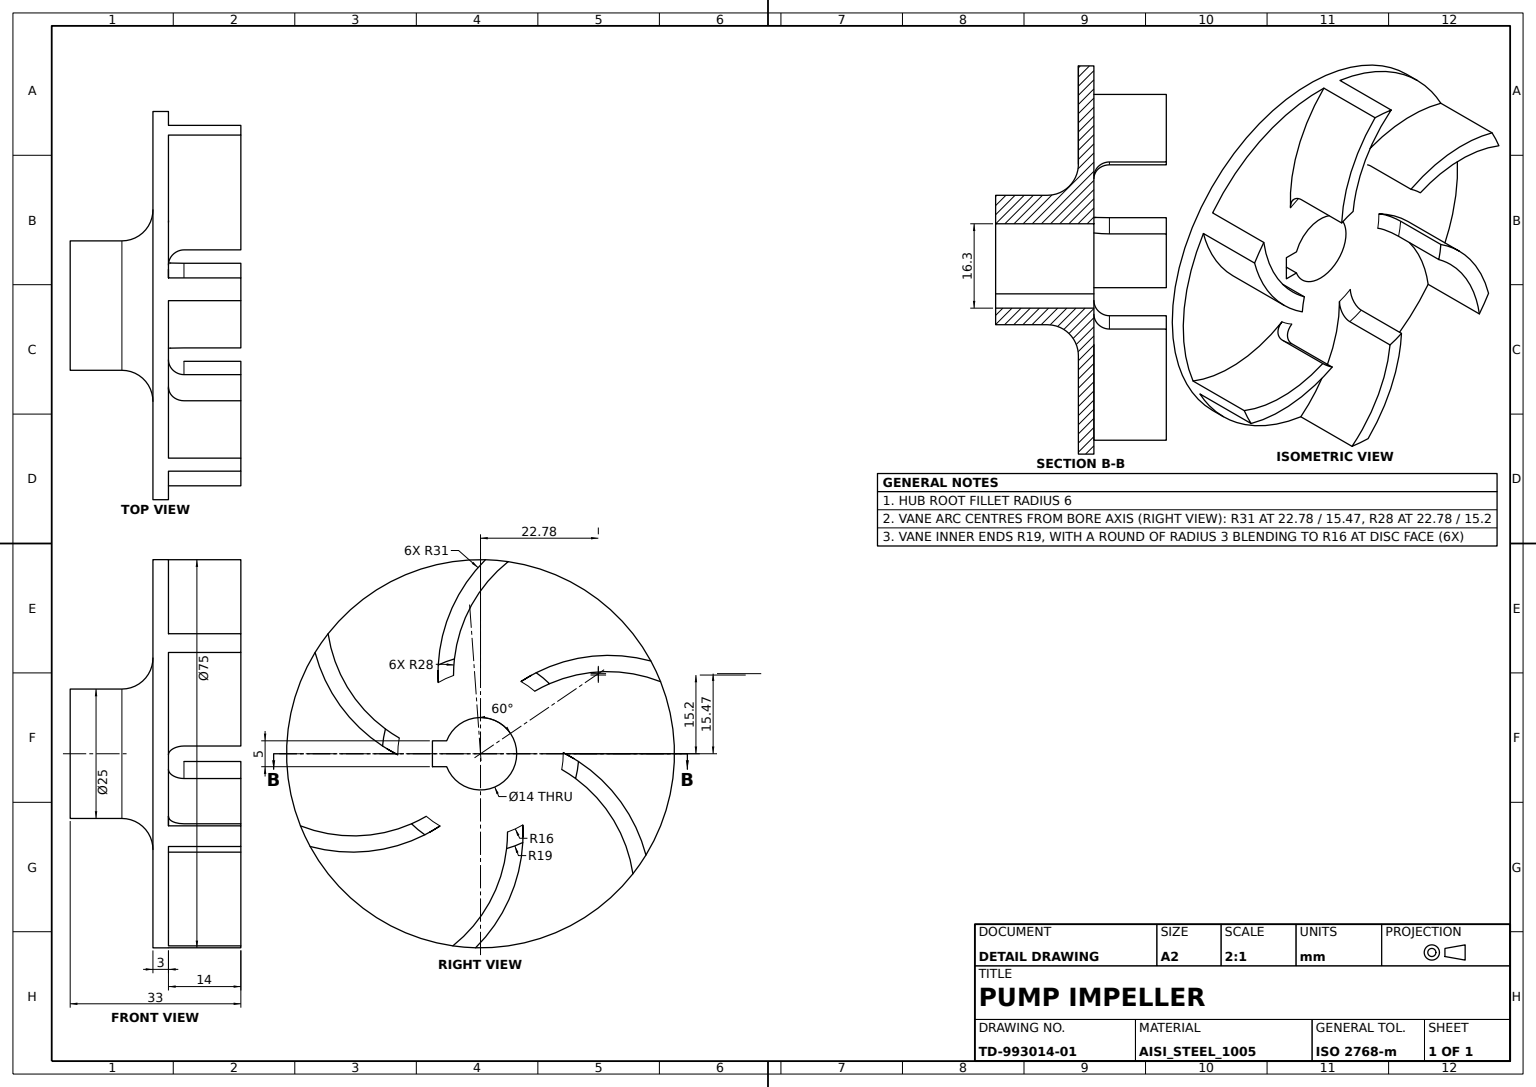
ISO-10303-21;
HEADER;
FILE_DESCRIPTION((''),'2;1');
FILE_NAME('','',(''),(''),'','','');
FILE_SCHEMA(('AUTOMOTIVE_DESIGN'));
ENDSEC;
DATA;
#1=APPLICATION_CONTEXT('');
#2=PRODUCT_CONTEXT('',#1,'mechanical');
#3=PRODUCT('','','',(#2));
#4=PRODUCT_DEFINITION_FORMATION('','',#3);
#5=PRODUCT_DEFINITION_CONTEXT('',#1,'design');
#6=PRODUCT_DEFINITION('','',#4,#5);
#7=PRODUCT_DEFINITION_SHAPE('','',#6);
#8=(LENGTH_UNIT()NAMED_UNIT(*)SI_UNIT(.MILLI.,.METRE.));
#9=(NAMED_UNIT(*)PLANE_ANGLE_UNIT()SI_UNIT($,.RADIAN.));
#10=(NAMED_UNIT(*)SI_UNIT($,.STERADIAN.)SOLID_ANGLE_UNIT());
#11=UNCERTAINTY_MEASURE_WITH_UNIT(LENGTH_MEASURE(0.005),#8,'distance_accuracy_value','');
#12=(GEOMETRIC_REPRESENTATION_CONTEXT(3)GLOBAL_UNCERTAINTY_ASSIGNED_CONTEXT((#11))GLOBAL_UNIT_ASSIGNED_CONTEXT((#8,#9,#10))REPRESENTATION_CONTEXT('',''));
#13=CARTESIAN_POINT('',(13.955798,-7.825324,3.));
#14=VERTEX_POINT('',#13);
#15=CARTESIAN_POINT('',(15.655908,-10.76534,6.));
#16=VERTEX_POINT('',#15);
#17=CARTESIAN_POINT('',(14.418426,-8.532847,3.));
#18=CARTESIAN_POINT('',(15.269698,-9.982915,3.553087));
#19=CARTESIAN_POINT('',(15.655908,-10.76534,5.151041));
#20=B_SPLINE_CURVE_WITH_KNOTS('',3,(#13,#17,#18,#19,#15),.UNSPECIFIED.,.F.,.F.,(4,1,4),(0.,0.002500889,0.005001779),.UNSPECIFIED.);
#21=EDGE_CURVE('',#14,#16,#20,.T.);
#22=ORIENTED_EDGE('',*,*,#21,.F.);
#23=CARTESIAN_POINT('',(12.083624,-10.487423,3.));
#24=VERTEX_POINT('',#23);
#25=CARTESIAN_POINT('',(0.,0.,3.));
#26=DIRECTION('',(0.,0.,-1.));
#27=DIRECTION('',(-1.,0.,0.));
#28=AXIS2_PLACEMENT_3D('',#25,#26,#27);
#29=CIRCLE('',#28,16.);
#30=EDGE_CURVE('',#24,#14,#29,.F.);
#31=ORIENTED_EDGE('',*,*,#30,.F.);
#32=CARTESIAN_POINT('',(13.529978,-13.339404,6.));
#33=VERTEX_POINT('',#32);
#34=CARTESIAN_POINT('',(13.529978,-13.339404,5.18123));
#35=CARTESIAN_POINT('',(13.234606,-12.637264,3.606546));
#36=CARTESIAN_POINT('',(12.494395,-11.194193,3.));
#37=B_SPLINE_CURVE_WITH_KNOTS('',3,(#32,#34,#35,#36,#23),.UNSPECIFIED.,.F.,.F.,(4,1,4),(0.,0.002420193,0.004840386),.UNSPECIFIED.);
#38=EDGE_CURVE('',#33,#24,#37,.T.);
#39=ORIENTED_EDGE('',*,*,#38,.F.);
#40=CARTESIAN_POINT('',(0.,0.,6.));
#41=AXIS2_PLACEMENT_3D('',#40,#26,#27);
#42=CIRCLE('',#41,19.);
#43=EDGE_CURVE('',#16,#33,#42,.T.);
#44=ORIENTED_EDGE('',*,*,#43,.F.);
#45=EDGE_LOOP('',(#22,#31,#39,#44));
#46=FACE_BOUND('',#45,.T.);
#47=TOROIDAL_SURFACE('',#41,16.,3.);
#48=ADVANCED_FACE('',(#46),#47,.F.);
#49=CARTESIAN_POINT('',(-23.189211,-29.470502,17.));
#50=VERTEX_POINT('',#49);
#51=CARTESIAN_POINT('',(-4.787274,-18.387006,17.));
#52=VERTEX_POINT('',#51);
#53=CARTESIAN_POINT('',(-27.329474,-1.778297,17.));
#54=DIRECTION('',(0.,0.,1.));
#55=DIRECTION('',(0.5,0.866025404,0.));
#56=AXIS2_PLACEMENT_3D('',#53,#54,#55);
#57=CIRCLE('',#56,28.);
#58=EDGE_CURVE('',#50,#52,#57,.T.);
#59=ORIENTED_EDGE('',*,*,#58,.F.);
#60=CARTESIAN_POINT('',(-19.568753,-31.989278,17.));
#61=VERTEX_POINT('',#60);
#62=CARTESIAN_POINT('',(0.,0.,17.));
#63=DIRECTION('',(1.,0.,0.));
#64=AXIS2_PLACEMENT_3D('',#62,#26,#63);
#65=CIRCLE('',#64,37.5);
#66=EDGE_CURVE('',#61,#50,#65,.T.);
#67=ORIENTED_EDGE('',*,*,#66,.F.);
#68=CARTESIAN_POINT('',(-1.495104,-18.941084,17.));
#69=VERTEX_POINT('',#68);
#70=CARTESIAN_POINT('',(-27.464158,-2.011577,17.));
#71=AXIS2_PLACEMENT_3D('',#70,#26,#55);
#72=CIRCLE('',#71,31.);
#73=EDGE_CURVE('',#69,#61,#72,.T.);
#74=ORIENTED_EDGE('',*,*,#73,.F.);
#75=AXIS2_PLACEMENT_3D('',#62,#54,#55);
#76=CIRCLE('',#75,19.);
#77=EDGE_CURVE('',#52,#69,#76,.T.);
#78=ORIENTED_EDGE('',*,*,#77,.F.);
#79=EDGE_LOOP('',(#59,#67,#74,#78));
#80=FACE_BOUND('',#79,.T.);
#81=CARTESIAN_POINT('',(-13.664737,-0.889148,17.));
#82=AXIS2_PLACEMENT_3D('',#81,#54,#63);
#83=PLANE('',#82);
#84=ADVANCED_FACE('',(#80),#83,.T.);
#85=CARTESIAN_POINT('',(0.20097,-15.998738,3.));
#86=VERTEX_POINT('',#85);
#87=CARTESIAN_POINT('',(-1.495104,-18.941084,6.));
#88=VERTEX_POINT('',#87);
#89=CARTESIAN_POINT('',(-0.18045,-16.753147,3.));
#90=CARTESIAN_POINT('',(-1.010609,-18.215404,3.553087));
#91=CARTESIAN_POINT('',(-1.495104,-18.941084,5.151041));
#92=B_SPLINE_CURVE_WITH_KNOTS('',3,(#85,#89,#90,#91,#87),.UNSPECIFIED.,.F.,.F.,(4,1,4),(0.,0.002500889,0.005001779),.UNSPECIFIED.);
#93=EDGE_CURVE('',#86,#88,#92,.T.);
#94=ORIENTED_EDGE('',*,*,#93,.F.);
#95=CARTESIAN_POINT('',(-3.040563,-15.708437,3.));
#96=VERTEX_POINT('',#95);
#97=EDGE_CURVE('',#96,#86,#29,.F.);
#98=ORIENTED_EDGE('',*,*,#97,.F.);
#99=CARTESIAN_POINT('',(-4.787274,-18.387006,6.));
#100=VERTEX_POINT('',#99);
#101=CARTESIAN_POINT('',(-4.787274,-18.387006,5.18123));
#102=CARTESIAN_POINT('',(-4.326889,-17.780137,3.606546));
#103=CARTESIAN_POINT('',(-3.447258,-16.41756,3.));
#104=B_SPLINE_CURVE_WITH_KNOTS('',3,(#99,#101,#102,#103,#95),.UNSPECIFIED.,.F.,.F.,(4,1,4),(0.,0.002420193,0.004840386),.UNSPECIFIED.);
#105=EDGE_CURVE('',#100,#96,#104,.T.);
#106=ORIENTED_EDGE('',*,*,#105,.F.);
#107=EDGE_CURVE('',#88,#100,#42,.T.);
#108=ORIENTED_EDGE('',*,*,#107,.F.);
#109=EDGE_LOOP('',(#94,#98,#106,#108));
#110=FACE_BOUND('',#109,.T.);
#111=ADVANCED_FACE('',(#110),#47,.F.);
#112=CARTESIAN_POINT('',(17.919151,-32.941676,3.));
#113=VERTEX_POINT('',#112);
#114=CARTESIAN_POINT('',(-11.990002,-24.790447,3.));
#115=DIRECTION('',(-0.5,0.866025404,0.));
#116=AXIS2_PLACEMENT_3D('',#114,#54,#115);
#117=CIRCLE('',#116,31.);
#118=EDGE_CURVE('',#113,#14,#117,.T.);
#119=ORIENTED_EDGE('',*,*,#118,.T.);
#120=ORIENTED_EDGE('',*,*,#21,.T.);
#121=CARTESIAN_POINT('',(15.655908,-10.76534,17.));
#122=VERTEX_POINT('',#121);
#123=VECTOR('',#26,1000.);
#124=LINE('',#121,#123);
#125=EDGE_CURVE('',#122,#16,#124,.T.);
#126=ORIENTED_EDGE('',*,*,#125,.F.);
#127=CARTESIAN_POINT('',(17.919151,-32.941676,17.));
#128=VERTEX_POINT('',#127);
#129=CARTESIAN_POINT('',(-11.990002,-24.790447,17.));
#130=AXIS2_PLACEMENT_3D('',#129,#54,#115);
#131=CIRCLE('',#130,31.);
#132=EDGE_CURVE('',#128,#122,#131,.T.);
#133=ORIENTED_EDGE('',*,*,#132,.F.);
#134=LINE('',#127,#123);
#135=EDGE_CURVE('',#128,#113,#134,.T.);
#136=ORIENTED_EDGE('',*,*,#135,.T.);
#137=EDGE_LOOP('',(#119,#120,#126,#133,#136));
#138=FACE_BOUND('',#137,.T.);
#139=AXIS2_PLACEMENT_3D('',#129,#26,#27);
#140=CYLINDRICAL_SURFACE('',#139,31.);
#141=ADVANCED_FACE('',(#138),#140,.T.);
#142=CARTESIAN_POINT('',(-17.151012,-8.175744,6.));
#143=VERTEX_POINT('',#142);
#144=CARTESIAN_POINT('',(-18.317252,-5.047602,6.));
#145=VERTEX_POINT('',#144);
#146=EDGE_CURVE('',#143,#145,#42,.T.);
#147=ORIENTED_EDGE('',*,*,#146,.T.);
#148=CARTESIAN_POINT('',(-18.317252,-5.047602,17.));
#149=VERTEX_POINT('',#148);
#150=LINE('',#148,#123);
#151=EDGE_CURVE('',#149,#145,#150,.T.);
#152=ORIENTED_EDGE('',*,*,#151,.F.);
#153=CARTESIAN_POINT('',(-17.151012,-8.175744,17.));
#154=VERTEX_POINT('',#153);
#155=AXIS2_PLACEMENT_3D('',#62,#54,#63);
#156=CIRCLE('',#155,19.);
#157=EDGE_CURVE('',#149,#154,#156,.T.);
#158=ORIENTED_EDGE('',*,*,#157,.T.);
#159=LINE('',#153,#123);
#160=EDGE_CURVE('',#154,#143,#159,.T.);
#161=ORIENTED_EDGE('',*,*,#160,.T.);
#162=EDGE_LOOP('',(#147,#152,#158,#161));
#163=FACE_BOUND('',#162,.T.);
#164=AXIS2_PLACEMENT_3D('',#62,#26,#27);
#165=CYLINDRICAL_SURFACE('',#164,19.);
#166=ADVANCED_FACE('',(#163),#165,.F.);
#167=CARTESIAN_POINT('',(2.5,-9.3,3.));
#168=VERTEX_POINT('',#167);
#169=CARTESIAN_POINT('',(2.5,-6.538348,3.));
#170=VERTEX_POINT('',#169);
#171=CARTESIAN_POINT('',(2.5,0.,3.));
#172=DIRECTION('',(0.,1.,0.));
#173=VECTOR('',#172,1000.);
#174=LINE('',#171,#173);
#175=EDGE_CURVE('',#168,#170,#174,.T.);
#176=ORIENTED_EDGE('',*,*,#175,.F.);
#177=CARTESIAN_POINT('',(-2.5,-9.3,3.));
#178=VERTEX_POINT('',#177);
#179=CARTESIAN_POINT('',(0.,-9.3,3.));
#180=VECTOR('',#63,1000.);
#181=LINE('',#179,#180);
#182=EDGE_CURVE('',#178,#168,#181,.T.);
#183=ORIENTED_EDGE('',*,*,#182,.F.);
#184=CARTESIAN_POINT('',(-2.5,-6.538348,3.));
#185=VERTEX_POINT('',#184);
#186=CARTESIAN_POINT('',(-2.5,0.,3.));
#187=DIRECTION('',(0.,-1.,0.));
#188=VECTOR('',#187,1000.);
#189=LINE('',#186,#188);
#190=EDGE_CURVE('',#185,#178,#189,.T.);
#191=ORIENTED_EDGE('',*,*,#190,.F.);
#192=CIRCLE('',#28,7.);
#193=EDGE_CURVE('',#170,#185,#192,.F.);
#194=ORIENTED_EDGE('',*,*,#193,.F.);
#195=EDGE_LOOP('',(#176,#183,#191,#194));
#196=FACE_BOUND('',#195,.T.);
#197=CARTESIAN_POINT('',(-23.189211,-29.470502,3.));
#198=VERTEX_POINT('',#197);
#199=CARTESIAN_POINT('',(-37.487904,0.952398,3.));
#200=VERTEX_POINT('',#199);
#201=AXIS2_PLACEMENT_3D('',#25,#26,#63);
#202=CIRCLE('',#201,37.5);
#203=EDGE_CURVE('',#198,#200,#202,.T.);
#204=ORIENTED_EDGE('',*,*,#203,.F.);
#205=CARTESIAN_POINT('',(-27.329474,-1.778297,3.));
#206=AXIS2_PLACEMENT_3D('',#205,#54,#55);
#207=CIRCLE('',#206,28.);
#208=EDGE_CURVE('',#198,#96,#207,.T.);
#209=ORIENTED_EDGE('',*,*,#208,.T.);
#210=ORIENTED_EDGE('',*,*,#97,.T.);
#211=CARTESIAN_POINT('',(-19.568753,-31.989278,3.));
#212=VERTEX_POINT('',#211);
#213=CARTESIAN_POINT('',(-27.464158,-2.011577,3.));
#214=AXIS2_PLACEMENT_3D('',#213,#26,#55);
#215=CIRCLE('',#214,31.);
#216=EDGE_CURVE('',#86,#212,#215,.T.);
#217=ORIENTED_EDGE('',*,*,#216,.T.);
#218=CARTESIAN_POINT('',(13.927598,-34.817697,3.));
#219=VERTEX_POINT('',#218);
#220=EDGE_CURVE('',#219,#212,#202,.T.);
#221=ORIENTED_EDGE('',*,*,#220,.F.);
#222=CARTESIAN_POINT('',(-12.124687,-24.557167,3.));
#223=AXIS2_PLACEMENT_3D('',#222,#26,#115);
#224=CIRCLE('',#223,28.);
#225=EDGE_CURVE('',#24,#219,#224,.T.);
#226=ORIENTED_EDGE('',*,*,#225,.F.);
#227=ORIENTED_EDGE('',*,*,#30,.T.);
#228=ORIENTED_EDGE('',*,*,#118,.F.);
#229=CARTESIAN_POINT('',(37.116809,-5.347195,3.));
#230=VERTEX_POINT('',#229);
#231=EDGE_CURVE('',#230,#113,#202,.T.);
#232=ORIENTED_EDGE('',*,*,#231,.F.);
#233=CARTESIAN_POINT('',(15.124186,5.221014,3.));
#234=VERTEX_POINT('',#233);
#235=CARTESIAN_POINT('',(15.204787,-22.77887,3.));
#236=AXIS2_PLACEMENT_3D('',#235,#26,#27);
#237=CIRCLE('',#236,28.);
#238=EDGE_CURVE('',#234,#230,#237,.T.);
#239=ORIENTED_EDGE('',*,*,#238,.F.);
#240=CARTESIAN_POINT('',(13.754828,8.173414,3.));
#241=VERTEX_POINT('',#240);
#242=EDGE_CURVE('',#234,#241,#29,.F.);
#243=ORIENTED_EDGE('',*,*,#242,.T.);
#244=CARTESIAN_POINT('',(37.487904,-0.952398,3.));
#245=VERTEX_POINT('',#244);
#246=CARTESIAN_POINT('',(15.474156,-22.77887,3.));
#247=AXIS2_PLACEMENT_3D('',#246,#54,#27);
#248=CIRCLE('',#247,31.);
#249=EDGE_CURVE('',#245,#241,#248,.T.);
#250=ORIENTED_EDGE('',*,*,#249,.F.);
#251=CARTESIAN_POINT('',(23.189211,29.470502,3.));
#252=VERTEX_POINT('',#251);
#253=EDGE_CURVE('',#252,#245,#202,.T.);
#254=ORIENTED_EDGE('',*,*,#253,.F.);
#255=CARTESIAN_POINT('',(3.040563,15.708437,3.));
#256=VERTEX_POINT('',#255);
#257=CARTESIAN_POINT('',(27.329474,1.778297,3.));
#258=DIRECTION('',(-0.5,-0.866025404,0.));
#259=AXIS2_PLACEMENT_3D('',#257,#26,#258);
#260=CIRCLE('',#259,28.);
#261=EDGE_CURVE('',#256,#252,#260,.T.);
#262=ORIENTED_EDGE('',*,*,#261,.F.);
#263=CARTESIAN_POINT('',(-0.20097,15.998738,3.));
#264=VERTEX_POINT('',#263);
#265=EDGE_CURVE('',#256,#264,#29,.F.);
#266=ORIENTED_EDGE('',*,*,#265,.T.);
#267=CARTESIAN_POINT('',(19.568753,31.989278,3.));
#268=VERTEX_POINT('',#267);
#269=CARTESIAN_POINT('',(27.464158,2.011577,3.));
#270=AXIS2_PLACEMENT_3D('',#269,#54,#258);
#271=CIRCLE('',#270,31.);
#272=EDGE_CURVE('',#268,#264,#271,.T.);
#273=ORIENTED_EDGE('',*,*,#272,.F.);
#274=CARTESIAN_POINT('',(-13.927598,34.817697,3.));
#275=VERTEX_POINT('',#274);
#276=EDGE_CURVE('',#275,#268,#202,.T.);
#277=ORIENTED_EDGE('',*,*,#276,.F.);
#278=CARTESIAN_POINT('',(-12.083624,10.487423,3.));
#279=VERTEX_POINT('',#278);
#280=CARTESIAN_POINT('',(12.124687,24.557167,3.));
#281=DIRECTION('',(0.5,-0.866025404,0.));
#282=AXIS2_PLACEMENT_3D('',#280,#54,#281);
#283=CIRCLE('',#282,28.);
#284=EDGE_CURVE('',#275,#279,#283,.T.);
#285=ORIENTED_EDGE('',*,*,#284,.T.);
#286=CARTESIAN_POINT('',(-13.955798,7.825324,3.));
#287=VERTEX_POINT('',#286);
#288=EDGE_CURVE('',#279,#287,#29,.F.);
#289=ORIENTED_EDGE('',*,*,#288,.T.);
#290=CARTESIAN_POINT('',(-17.919151,32.941676,3.));
#291=VERTEX_POINT('',#290);
#292=CARTESIAN_POINT('',(11.990002,24.790447,3.));
#293=AXIS2_PLACEMENT_3D('',#292,#26,#281);
#294=CIRCLE('',#293,31.);
#295=EDGE_CURVE('',#287,#291,#294,.T.);
#296=ORIENTED_EDGE('',*,*,#295,.T.);
#297=CARTESIAN_POINT('',(-37.116809,5.347195,3.));
#298=VERTEX_POINT('',#297);
#299=EDGE_CURVE('',#298,#291,#202,.T.);
#300=ORIENTED_EDGE('',*,*,#299,.F.);
#301=CARTESIAN_POINT('',(-15.124186,-5.221014,3.));
#302=VERTEX_POINT('',#301);
#303=CARTESIAN_POINT('',(-15.204787,22.77887,3.));
#304=AXIS2_PLACEMENT_3D('',#303,#54,#63);
#305=CIRCLE('',#304,28.);
#306=EDGE_CURVE('',#298,#302,#305,.T.);
#307=ORIENTED_EDGE('',*,*,#306,.T.);
#308=CARTESIAN_POINT('',(-13.754828,-8.173414,3.));
#309=VERTEX_POINT('',#308);
#310=EDGE_CURVE('',#302,#309,#29,.F.);
#311=ORIENTED_EDGE('',*,*,#310,.T.);
#312=CARTESIAN_POINT('',(-15.474156,22.77887,3.));
#313=AXIS2_PLACEMENT_3D('',#312,#26,#63);
#314=CIRCLE('',#313,31.);
#315=EDGE_CURVE('',#309,#200,#314,.T.);
#316=ORIENTED_EDGE('',*,*,#315,.T.);
#317=EDGE_LOOP('',(#204,#209,#210,#217,#221,#226,#227,#228,#232,#239,#243,#250,#254,#262,#266,#273,#277,#285,#289,#296,#300,#307,#311,#316));
#318=FACE_BOUND('',#317,.T.);
#319=PLANE('',#28);
#320=ADVANCED_FACE('',(#196,#318),#319,.F.);
#321=ORIENTED_EDGE('',*,*,#272,.T.);
#322=CARTESIAN_POINT('',(1.495104,18.941084,6.));
#323=VERTEX_POINT('',#322);
#324=CARTESIAN_POINT('',(0.18045,16.753147,3.));
#325=CARTESIAN_POINT('',(1.010609,18.215404,3.553087));
#326=CARTESIAN_POINT('',(1.495104,18.941084,5.151041));
#327=B_SPLINE_CURVE_WITH_KNOTS('',3,(#263,#324,#325,#326,#322),.UNSPECIFIED.,.F.,.F.,(4,1,4),(0.,0.002500889,0.005001779),.UNSPECIFIED.);
#328=EDGE_CURVE('',#264,#323,#327,.T.);
#329=ORIENTED_EDGE('',*,*,#328,.T.);
#330=CARTESIAN_POINT('',(1.495104,18.941084,17.));
#331=VERTEX_POINT('',#330);
#332=LINE('',#330,#123);
#333=EDGE_CURVE('',#331,#323,#332,.T.);
#334=ORIENTED_EDGE('',*,*,#333,.F.);
#335=CARTESIAN_POINT('',(19.568753,31.989278,17.));
#336=VERTEX_POINT('',#335);
#337=CARTESIAN_POINT('',(27.464158,2.011577,17.));
#338=AXIS2_PLACEMENT_3D('',#337,#54,#258);
#339=CIRCLE('',#338,31.);
#340=EDGE_CURVE('',#336,#331,#339,.T.);
#341=ORIENTED_EDGE('',*,*,#340,.F.);
#342=LINE('',#335,#123);
#343=EDGE_CURVE('',#336,#268,#342,.T.);
#344=ORIENTED_EDGE('',*,*,#343,.T.);
#345=EDGE_LOOP('',(#321,#329,#334,#341,#344));
#346=FACE_BOUND('',#345,.T.);
#347=AXIS2_PLACEMENT_3D('',#337,#26,#27);
#348=CYLINDRICAL_SURFACE('',#347,31.);
#349=ADVANCED_FACE('',(#346),#348,.T.);
#350=CARTESIAN_POINT('',(17.151012,8.175744,17.));
#351=VERTEX_POINT('',#350);
#352=CARTESIAN_POINT('',(17.151012,8.175744,6.));
#353=VERTEX_POINT('',#352);
#354=LINE('',#350,#123);
#355=EDGE_CURVE('',#351,#353,#354,.T.);
#356=ORIENTED_EDGE('',*,*,#355,.T.);
#357=CARTESIAN_POINT('',(18.317252,5.047602,6.));
#358=VERTEX_POINT('',#357);
#359=EDGE_CURVE('',#353,#358,#42,.T.);
#360=ORIENTED_EDGE('',*,*,#359,.T.);
#361=CARTESIAN_POINT('',(18.317252,5.047602,17.));
#362=VERTEX_POINT('',#361);
#363=LINE('',#361,#123);
#364=EDGE_CURVE('',#362,#358,#363,.T.);
#365=ORIENTED_EDGE('',*,*,#364,.F.);
#366=CIRCLE('',#164,19.);
#367=EDGE_CURVE('',#351,#362,#366,.T.);
#368=ORIENTED_EDGE('',*,*,#367,.F.);
#369=EDGE_LOOP('',(#356,#360,#365,#368));
#370=FACE_BOUND('',#369,.T.);
#371=ADVANCED_FACE('',(#370),#165,.F.);
#372=CARTESIAN_POINT('',(-2.5,-9.3,-16.));
#373=VERTEX_POINT('',#372);
#374=CARTESIAN_POINT('',(2.5,-9.3,-16.));
#375=VERTEX_POINT('',#374);
#376=LINE('',#372,#180);
#377=EDGE_CURVE('',#373,#375,#376,.T.);
#378=ORIENTED_EDGE('',*,*,#377,.T.);
#379=CARTESIAN_POINT('',(2.5,-6.538348,-16.));
#380=VERTEX_POINT('',#379);
#381=LINE('',#374,#173);
#382=EDGE_CURVE('',#375,#380,#381,.T.);
#383=ORIENTED_EDGE('',*,*,#382,.T.);
#384=CARTESIAN_POINT('',(-2.5,-6.538348,-16.));
#385=VERTEX_POINT('',#384);
#386=CARTESIAN_POINT('',(0.,0.,-16.));
#387=AXIS2_PLACEMENT_3D('',#386,#54,#63);
#388=CIRCLE('',#387,7.);
#389=EDGE_CURVE('',#380,#385,#388,.T.);
#390=ORIENTED_EDGE('',*,*,#389,.T.);
#391=LINE('',#384,#188);
#392=EDGE_CURVE('',#385,#373,#391,.T.);
#393=ORIENTED_EDGE('',*,*,#392,.T.);
#394=EDGE_LOOP('',(#378,#383,#390,#393));
#395=FACE_BOUND('',#394,.T.);
#396=CARTESIAN_POINT('',(12.5,0.,-16.));
#397=VERTEX_POINT('',#396);
#398=AXIS2_PLACEMENT_3D('',#386,#26,#63);
#399=CIRCLE('',#398,12.5);
#400=EDGE_CURVE('',#397,#397,#399,.T.);
#401=ORIENTED_EDGE('',*,*,#400,.T.);
#402=EDGE_LOOP('',(#401));
#403=FACE_BOUND('',#402,.T.);
#404=AXIS2_PLACEMENT_3D('',#386,#26,#27);
#405=PLANE('',#404);
#406=ADVANCED_FACE('',(#395,#403),#405,.T.);
#407=CARTESIAN_POINT('',(13.529978,-13.339404,17.));
#408=VERTEX_POINT('',#407);
#409=LINE('',#407,#123);
#410=EDGE_CURVE('',#408,#33,#409,.T.);
#411=ORIENTED_EDGE('',*,*,#410,.F.);
#412=AXIS2_PLACEMENT_3D('',#62,#26,#115);
#413=CIRCLE('',#412,19.);
#414=EDGE_CURVE('',#122,#408,#413,.T.);
#415=ORIENTED_EDGE('',*,*,#414,.F.);
#416=ORIENTED_EDGE('',*,*,#125,.T.);
#417=ORIENTED_EDGE('',*,*,#43,.T.);
#418=EDGE_LOOP('',(#411,#415,#416,#417));
#419=FACE_BOUND('',#418,.T.);
#420=ADVANCED_FACE('',(#419),#165,.F.);
#421=LINE('',#49,#123);
#422=EDGE_CURVE('',#50,#198,#421,.T.);
#423=ORIENTED_EDGE('',*,*,#422,.F.);
#424=ORIENTED_EDGE('',*,*,#58,.T.);
#425=LINE('',#51,#123);
#426=EDGE_CURVE('',#52,#100,#425,.T.);
#427=ORIENTED_EDGE('',*,*,#426,.T.);
#428=ORIENTED_EDGE('',*,*,#105,.T.);
#429=ORIENTED_EDGE('',*,*,#208,.F.);
#430=EDGE_LOOP('',(#423,#424,#427,#428,#429));
#431=FACE_BOUND('',#430,.T.);
#432=AXIS2_PLACEMENT_3D('',#53,#26,#27);
#433=CYLINDRICAL_SURFACE('',#432,28.);
#434=ADVANCED_FACE('',(#431),#433,.F.);
#435=CARTESIAN_POINT('',(13.927598,-34.817697,17.));
#436=VERTEX_POINT('',#435);
#437=LINE('',#435,#123);
#438=EDGE_CURVE('',#436,#219,#437,.T.);
#439=ORIENTED_EDGE('',*,*,#438,.F.);
#440=CARTESIAN_POINT('',(-12.124687,-24.557167,17.));
#441=AXIS2_PLACEMENT_3D('',#440,#26,#115);
#442=CIRCLE('',#441,28.);
#443=EDGE_CURVE('',#408,#436,#442,.T.);
#444=ORIENTED_EDGE('',*,*,#443,.F.);
#445=ORIENTED_EDGE('',*,*,#410,.T.);
#446=ORIENTED_EDGE('',*,*,#38,.T.);
#447=ORIENTED_EDGE('',*,*,#225,.T.);
#448=EDGE_LOOP('',(#439,#444,#445,#446,#447));
#449=FACE_BOUND('',#448,.T.);
#450=AXIS2_PLACEMENT_3D('',#440,#26,#27);
#451=CYLINDRICAL_SURFACE('',#450,28.);
#452=ADVANCED_FACE('',(#449),#451,.F.);
#453=CARTESIAN_POINT('',(2.5,-9.3,14.));
#454=LINE('',#453,#123);
#455=EDGE_CURVE('',#375,#168,#454,.F.);
#456=ORIENTED_EDGE('',*,*,#455,.T.);
#457=ORIENTED_EDGE('',*,*,#175,.T.);
#458=CARTESIAN_POINT('',(2.5,-6.538348,14.));
#459=LINE('',#458,#123);
#460=EDGE_CURVE('',#380,#170,#459,.F.);
#461=ORIENTED_EDGE('',*,*,#460,.F.);
#462=ORIENTED_EDGE('',*,*,#382,.F.);
#463=EDGE_LOOP('',(#456,#457,#461,#462));
#464=FACE_BOUND('',#463,.T.);
#465=AXIS2_PLACEMENT_3D('',#453,#27,#187);
#466=PLANE('',#465);
#467=ADVANCED_FACE('',(#464),#466,.T.);
#468=ORIENTED_EDGE('',*,*,#426,.F.);
#469=ORIENTED_EDGE('',*,*,#77,.T.);
#470=LINE('',#68,#123);
#471=EDGE_CURVE('',#69,#88,#470,.T.);
#472=ORIENTED_EDGE('',*,*,#471,.T.);
#473=ORIENTED_EDGE('',*,*,#107,.T.);
#474=EDGE_LOOP('',(#468,#469,#472,#473));
#475=FACE_BOUND('',#474,.T.);
#476=ADVANCED_FACE('',(#475),#165,.F.);
#477=CARTESIAN_POINT('',(-14.598875,-8.220299,3.));
#478=CARTESIAN_POINT('',(-16.280307,-8.232489,3.553087));
#479=CARTESIAN_POINT('',(-17.151012,-8.175744,5.151041));
#480=B_SPLINE_CURVE_WITH_KNOTS('',3,(#308,#477,#478,#479,#142),.UNSPECIFIED.,.F.,.F.,(4,1,4),(0.,0.002500889,0.005001779),.UNSPECIFIED.);
#481=EDGE_CURVE('',#309,#143,#480,.T.);
#482=ORIENTED_EDGE('',*,*,#481,.T.);
#483=ORIENTED_EDGE('',*,*,#160,.F.);
#484=CARTESIAN_POINT('',(-37.487904,0.952398,17.));
#485=VERTEX_POINT('',#484);
#486=CARTESIAN_POINT('',(-15.474156,22.77887,17.));
#487=AXIS2_PLACEMENT_3D('',#486,#26,#63);
#488=CIRCLE('',#487,31.);
#489=EDGE_CURVE('',#154,#485,#488,.T.);
#490=ORIENTED_EDGE('',*,*,#489,.T.);
#491=LINE('',#484,#123);
#492=EDGE_CURVE('',#485,#200,#491,.T.);
#493=ORIENTED_EDGE('',*,*,#492,.T.);
#494=ORIENTED_EDGE('',*,*,#315,.F.);
#495=EDGE_LOOP('',(#482,#483,#490,#493,#494));
#496=FACE_BOUND('',#495,.T.);
#497=AXIS2_PLACEMENT_3D('',#486,#26,#27);
#498=CYLINDRICAL_SURFACE('',#497,31.);
#499=ADVANCED_FACE('',(#496),#498,.T.);
#500=CARTESIAN_POINT('',(23.189211,29.470502,17.));
#501=VERTEX_POINT('',#500);
#502=LINE('',#500,#123);
#503=EDGE_CURVE('',#501,#252,#502,.T.);
#504=ORIENTED_EDGE('',*,*,#503,.F.);
#505=CARTESIAN_POINT('',(4.787274,18.387006,17.));
#506=VERTEX_POINT('',#505);
#507=CARTESIAN_POINT('',(27.329474,1.778297,17.));
#508=AXIS2_PLACEMENT_3D('',#507,#26,#258);
#509=CIRCLE('',#508,28.);
#510=EDGE_CURVE('',#506,#501,#509,.T.);
#511=ORIENTED_EDGE('',*,*,#510,.F.);
#512=CARTESIAN_POINT('',(4.787274,18.387006,6.));
#513=VERTEX_POINT('',#512);
#514=LINE('',#505,#123);
#515=EDGE_CURVE('',#506,#513,#514,.T.);
#516=ORIENTED_EDGE('',*,*,#515,.T.);
#517=CARTESIAN_POINT('',(4.787274,18.387006,5.18123));
#518=CARTESIAN_POINT('',(4.326889,17.780137,3.606546));
#519=CARTESIAN_POINT('',(3.447258,16.41756,3.));
#520=B_SPLINE_CURVE_WITH_KNOTS('',3,(#512,#517,#518,#519,#255),.UNSPECIFIED.,.F.,.F.,(4,1,4),(0.,0.002420193,0.004840386),.UNSPECIFIED.);
#521=EDGE_CURVE('',#513,#256,#520,.T.);
#522=ORIENTED_EDGE('',*,*,#521,.T.);
#523=ORIENTED_EDGE('',*,*,#261,.T.);
#524=EDGE_LOOP('',(#504,#511,#516,#522,#523));
#525=FACE_BOUND('',#524,.T.);
#526=AXIS2_PLACEMENT_3D('',#507,#26,#27);
#527=CYLINDRICAL_SURFACE('',#526,28.);
#528=ADVANCED_FACE('',(#525),#527,.F.);
#529=CARTESIAN_POINT('',(37.116809,-5.347195,17.));
#530=VERTEX_POINT('',#529);
#531=CARTESIAN_POINT('',(15.204787,-22.77887,17.));
#532=AXIS2_PLACEMENT_3D('',#531,#26,#27);
#533=CIRCLE('',#532,28.);
#534=EDGE_CURVE('',#362,#530,#533,.T.);
#535=ORIENTED_EDGE('',*,*,#534,.F.);
#536=ORIENTED_EDGE('',*,*,#364,.T.);
#537=CARTESIAN_POINT('',(18.317252,5.047602,5.18123));
#538=CARTESIAN_POINT('',(17.561495,5.142873,3.606546));
#539=CARTESIAN_POINT('',(15.941653,5.223367,3.));
#540=B_SPLINE_CURVE_WITH_KNOTS('',3,(#357,#537,#538,#539,#233),.UNSPECIFIED.,.F.,.F.,(4,1,4),(0.,0.002420193,0.004840386),.UNSPECIFIED.);
#541=EDGE_CURVE('',#358,#234,#540,.T.);
#542=ORIENTED_EDGE('',*,*,#541,.T.);
#543=ORIENTED_EDGE('',*,*,#238,.T.);
#544=LINE('',#529,#123);
#545=EDGE_CURVE('',#530,#230,#544,.T.);
#546=ORIENTED_EDGE('',*,*,#545,.F.);
#547=EDGE_LOOP('',(#535,#536,#542,#543,#546));
#548=FACE_BOUND('',#547,.T.);
#549=CYLINDRICAL_SURFACE('',#532,28.);
#550=ADVANCED_FACE('',(#548),#549,.F.);
#551=EDGE_CURVE('',#323,#513,#42,.T.);
#552=ORIENTED_EDGE('',*,*,#551,.F.);
#553=ORIENTED_EDGE('',*,*,#328,.F.);
#554=ORIENTED_EDGE('',*,*,#265,.F.);
#555=ORIENTED_EDGE('',*,*,#521,.F.);
#556=EDGE_LOOP('',(#552,#553,#554,#555));
#557=FACE_BOUND('',#556,.T.);
#558=ADVANCED_FACE('',(#557),#47,.F.);
#559=CARTESIAN_POINT('',(37.487904,-0.952398,17.));
#560=VERTEX_POINT('',#559);
#561=CARTESIAN_POINT('',(15.474156,-22.77887,17.));
#562=AXIS2_PLACEMENT_3D('',#561,#54,#27);
#563=CIRCLE('',#562,31.);
#564=EDGE_CURVE('',#560,#351,#563,.T.);
#565=ORIENTED_EDGE('',*,*,#564,.T.);
#566=ORIENTED_EDGE('',*,*,#367,.T.);
#567=ORIENTED_EDGE('',*,*,#534,.T.);
#568=CIRCLE('',#155,37.5);
#569=EDGE_CURVE('',#530,#560,#568,.T.);
#570=ORIENTED_EDGE('',*,*,#569,.T.);
#571=EDGE_LOOP('',(#565,#566,#567,#570));
#572=FACE_BOUND('',#571,.T.);
#573=CARTESIAN_POINT('',(7.602393,-11.389435,17.));
#574=AXIS2_PLACEMENT_3D('',#573,#26,#27);
#575=PLANE('',#574);
#576=ADVANCED_FACE('',(#572),#575,.F.);
#577=CARTESIAN_POINT('',(-15.655908,10.76534,17.));
#578=VERTEX_POINT('',#577);
#579=CARTESIAN_POINT('',(-15.655908,10.76534,6.));
#580=VERTEX_POINT('',#579);
#581=LINE('',#577,#123);
#582=EDGE_CURVE('',#578,#580,#581,.T.);
#583=ORIENTED_EDGE('',*,*,#582,.T.);
#584=CARTESIAN_POINT('',(-13.529978,13.339404,6.));
#585=VERTEX_POINT('',#584);
#586=EDGE_CURVE('',#580,#585,#42,.T.);
#587=ORIENTED_EDGE('',*,*,#586,.T.);
#588=CARTESIAN_POINT('',(-13.529978,13.339404,17.));
#589=VERTEX_POINT('',#588);
#590=LINE('',#588,#123);
#591=EDGE_CURVE('',#589,#585,#590,.T.);
#592=ORIENTED_EDGE('',*,*,#591,.F.);
#593=AXIS2_PLACEMENT_3D('',#62,#54,#281);
#594=CIRCLE('',#593,19.);
#595=EDGE_CURVE('',#589,#578,#594,.T.);
#596=ORIENTED_EDGE('',*,*,#595,.T.);
#597=EDGE_LOOP('',(#583,#587,#592,#596));
#598=FACE_BOUND('',#597,.T.);
#599=ADVANCED_FACE('',(#598),#165,.F.);
#600=ORIENTED_EDGE('',*,*,#132,.T.);
#601=ORIENTED_EDGE('',*,*,#414,.T.);
#602=ORIENTED_EDGE('',*,*,#443,.T.);
#603=EDGE_CURVE('',#436,#128,#568,.T.);
#604=ORIENTED_EDGE('',*,*,#603,.T.);
#605=EDGE_LOOP('',(#600,#601,#602,#604));
#606=FACE_BOUND('',#605,.T.);
#607=CARTESIAN_POINT('',(-5.995001,-12.395224,17.));
#608=AXIS2_PLACEMENT_3D('',#607,#54,#63);
#609=PLANE('',#608);
#610=ADVANCED_FACE('',(#606),#609,.T.);
#611=ORIENTED_EDGE('',*,*,#306,.F.);
#612=CARTESIAN_POINT('',(-37.116809,5.347195,17.));
#613=VERTEX_POINT('',#612);
#614=LINE('',#612,#123);
#615=EDGE_CURVE('',#613,#298,#614,.T.);
#616=ORIENTED_EDGE('',*,*,#615,.F.);
#617=CARTESIAN_POINT('',(-15.204787,22.77887,17.));
#618=AXIS2_PLACEMENT_3D('',#617,#54,#63);
#619=CIRCLE('',#618,28.);
#620=EDGE_CURVE('',#613,#149,#619,.T.);
#621=ORIENTED_EDGE('',*,*,#620,.T.);
#622=ORIENTED_EDGE('',*,*,#151,.T.);
#623=CARTESIAN_POINT('',(-18.317252,-5.047602,5.18123));
#624=CARTESIAN_POINT('',(-17.561495,-5.142873,3.606546));
#625=CARTESIAN_POINT('',(-15.941653,-5.223367,3.));
#626=B_SPLINE_CURVE_WITH_KNOTS('',3,(#144,#623,#624,#625,#301),.UNSPECIFIED.,.F.,.F.,(4,1,4),(0.,0.002420193,0.004840386),.UNSPECIFIED.);
#627=EDGE_CURVE('',#145,#302,#626,.T.);
#628=ORIENTED_EDGE('',*,*,#627,.T.);
#629=EDGE_LOOP('',(#611,#616,#621,#622,#628));
#630=FACE_BOUND('',#629,.T.);
#631=AXIS2_PLACEMENT_3D('',#617,#26,#27);
#632=CYLINDRICAL_SURFACE('',#631,28.);
#633=ADVANCED_FACE('',(#630),#632,.F.);
#634=CARTESIAN_POINT('',(-2.5,-9.3,14.));
#635=LINE('',#634,#123);
#636=EDGE_CURVE('',#373,#178,#635,.F.);
#637=ORIENTED_EDGE('',*,*,#636,.T.);
#638=ORIENTED_EDGE('',*,*,#182,.T.);
#639=ORIENTED_EDGE('',*,*,#455,.F.);
#640=ORIENTED_EDGE('',*,*,#377,.F.);
#641=EDGE_LOOP('',(#637,#638,#639,#640));
#642=FACE_BOUND('',#641,.T.);
#643=AXIS2_PLACEMENT_3D('',#634,#172,#54);
#644=PLANE('',#643);
#645=ADVANCED_FACE('',(#642),#644,.T.);
#646=ORIENTED_EDGE('',*,*,#489,.F.);
#647=ORIENTED_EDGE('',*,*,#157,.F.);
#648=ORIENTED_EDGE('',*,*,#620,.F.);
#649=EDGE_CURVE('',#485,#613,#65,.T.);
#650=ORIENTED_EDGE('',*,*,#649,.F.);
#651=EDGE_LOOP('',(#646,#647,#648,#650));
#652=FACE_BOUND('',#651,.T.);
#653=CARTESIAN_POINT('',(-7.602393,11.389435,17.));
#654=AXIS2_PLACEMENT_3D('',#653,#54,#63);
#655=PLANE('',#654);
#656=ADVANCED_FACE('',(#652),#655,.T.);
#657=CARTESIAN_POINT('',(-2.5,-6.538348,14.));
#658=LINE('',#657,#123);
#659=EDGE_CURVE('',#385,#185,#658,.F.);
#660=ORIENTED_EDGE('',*,*,#659,.F.);
#661=ORIENTED_EDGE('',*,*,#389,.F.);
#662=ORIENTED_EDGE('',*,*,#460,.T.);
#663=ORIENTED_EDGE('',*,*,#193,.T.);
#664=EDGE_LOOP('',(#660,#661,#662,#663));
#665=FACE_BOUND('',#664,.T.);
#666=CARTESIAN_POINT('',(0.,0.,14.));
#667=AXIS2_PLACEMENT_3D('',#666,#26,#27);
#668=CYLINDRICAL_SURFACE('',#667,7.);
#669=ADVANCED_FACE('',(#665),#668,.F.);
#670=CARTESIAN_POINT('',(-17.919151,32.941676,17.));
#671=VERTEX_POINT('',#670);
#672=CARTESIAN_POINT('',(11.990002,24.790447,17.));
#673=AXIS2_PLACEMENT_3D('',#672,#26,#281);
#674=CIRCLE('',#673,31.);
#675=EDGE_CURVE('',#578,#671,#674,.T.);
#676=ORIENTED_EDGE('',*,*,#675,.T.);
#677=LINE('',#670,#123);
#678=EDGE_CURVE('',#671,#291,#677,.T.);
#679=ORIENTED_EDGE('',*,*,#678,.T.);
#680=ORIENTED_EDGE('',*,*,#295,.F.);
#681=CARTESIAN_POINT('',(-14.418426,8.532847,3.));
#682=CARTESIAN_POINT('',(-15.269698,9.982915,3.553087));
#683=CARTESIAN_POINT('',(-15.655908,10.76534,5.151041));
#684=B_SPLINE_CURVE_WITH_KNOTS('',3,(#286,#681,#682,#683,#579),.UNSPECIFIED.,.F.,.F.,(4,1,4),(0.,0.002500889,0.005001779),.UNSPECIFIED.);
#685=EDGE_CURVE('',#287,#580,#684,.T.);
#686=ORIENTED_EDGE('',*,*,#685,.T.);
#687=ORIENTED_EDGE('',*,*,#582,.F.);
#688=EDGE_LOOP('',(#676,#679,#680,#686,#687));
#689=FACE_BOUND('',#688,.T.);
#690=AXIS2_PLACEMENT_3D('',#672,#26,#27);
#691=CYLINDRICAL_SURFACE('',#690,31.);
#692=ADVANCED_FACE('',(#689),#691,.T.);
#693=CARTESIAN_POINT('',(-12.5,0.,-6.));
#694=VERTEX_POINT('',#693);
#695=CARTESIAN_POINT('',(0.,0.,-6.));
#696=AXIS2_PLACEMENT_3D('',#695,#26,#27);
#697=CIRCLE('',#696,12.5);
#698=EDGE_CURVE('',#694,#694,#697,.T.);
#699=ORIENTED_EDGE('',*,*,#698,.F.);
#700=EDGE_LOOP('',(#699));
#701=FACE_BOUND('',#700,.T.);
#702=CARTESIAN_POINT('',(-18.5,0.,0.));
#703=VERTEX_POINT('',#702);
#704=CARTESIAN_POINT('',(0.,0.,0.));
#705=AXIS2_PLACEMENT_3D('',#704,#26,#27);
#706=CIRCLE('',#705,18.5);
#707=EDGE_CURVE('',#703,#703,#706,.F.);
#708=ORIENTED_EDGE('',*,*,#707,.F.);
#709=EDGE_LOOP('',(#708));
#710=FACE_BOUND('',#709,.T.);
#711=TOROIDAL_SURFACE('',#696,18.5,6.);
#712=ADVANCED_FACE('',(#701,#710),#711,.F.);
#713=ORIENTED_EDGE('',*,*,#636,.F.);
#714=ORIENTED_EDGE('',*,*,#392,.F.);
#715=ORIENTED_EDGE('',*,*,#659,.T.);
#716=ORIENTED_EDGE('',*,*,#190,.T.);
#717=EDGE_LOOP('',(#713,#714,#715,#716));
#718=FACE_BOUND('',#717,.T.);
#719=AXIS2_PLACEMENT_3D('',#657,#63,#172);
#720=PLANE('',#719);
#721=ADVANCED_FACE('',(#718),#720,.T.);
#722=CARTESIAN_POINT('',(37.5,0.,0.));
#723=VERTEX_POINT('',#722);
#724=AXIS2_PLACEMENT_3D('',#704,#26,#63);
#725=CIRCLE('',#724,37.5);
#726=EDGE_CURVE('',#723,#723,#725,.T.);
#727=ORIENTED_EDGE('',*,*,#726,.T.);
#728=EDGE_LOOP('',(#727));
#729=FACE_BOUND('',#728,.T.);
#730=ORIENTED_EDGE('',*,*,#707,.T.);
#731=EDGE_LOOP('',(#730));
#732=FACE_BOUND('',#731,.T.);
#733=PLANE('',#705);
#734=ADVANCED_FACE('',(#729,#732),#733,.T.);
#735=ORIENTED_EDGE('',*,*,#400,.F.);
#736=EDGE_LOOP('',(#735));
#737=FACE_BOUND('',#736,.T.);
#738=ORIENTED_EDGE('',*,*,#698,.T.);
#739=EDGE_LOOP('',(#738));
#740=FACE_BOUND('',#739,.T.);
#741=CYLINDRICAL_SURFACE('',#387,12.5);
#742=ADVANCED_FACE('',(#737,#740),#741,.T.);
#743=ORIENTED_EDGE('',*,*,#510,.T.);
#744=EDGE_CURVE('',#501,#336,#568,.T.);
#745=ORIENTED_EDGE('',*,*,#744,.T.);
#746=ORIENTED_EDGE('',*,*,#340,.T.);
#747=AXIS2_PLACEMENT_3D('',#62,#26,#258);
#748=CIRCLE('',#747,19.);
#749=EDGE_CURVE('',#331,#506,#748,.T.);
#750=ORIENTED_EDGE('',*,*,#749,.T.);
#751=EDGE_LOOP('',(#743,#745,#746,#750));
#752=FACE_BOUND('',#751,.T.);
#753=CARTESIAN_POINT('',(13.732079,1.005788,17.));
#754=AXIS2_PLACEMENT_3D('',#753,#54,#63);
#755=PLANE('',#754);
#756=ADVANCED_FACE('',(#752),#755,.T.);
#757=CARTESIAN_POINT('',(-13.529978,13.339404,5.18123));
#758=CARTESIAN_POINT('',(-13.234606,12.637264,3.606546));
#759=CARTESIAN_POINT('',(-12.494395,11.194193,3.));
#760=B_SPLINE_CURVE_WITH_KNOTS('',3,(#584,#757,#758,#759,#278),.UNSPECIFIED.,.F.,.F.,(4,1,4),(0.,0.002420193,0.004840386),.UNSPECIFIED.);
#761=EDGE_CURVE('',#585,#279,#760,.T.);
#762=ORIENTED_EDGE('',*,*,#761,.T.);
#763=ORIENTED_EDGE('',*,*,#284,.F.);
#764=CARTESIAN_POINT('',(-13.927598,34.817697,17.));
#765=VERTEX_POINT('',#764);
#766=LINE('',#764,#123);
#767=EDGE_CURVE('',#765,#275,#766,.T.);
#768=ORIENTED_EDGE('',*,*,#767,.F.);
#769=CARTESIAN_POINT('',(12.124687,24.557167,17.));
#770=AXIS2_PLACEMENT_3D('',#769,#54,#281);
#771=CIRCLE('',#770,28.);
#772=EDGE_CURVE('',#765,#589,#771,.T.);
#773=ORIENTED_EDGE('',*,*,#772,.T.);
#774=ORIENTED_EDGE('',*,*,#591,.T.);
#775=EDGE_LOOP('',(#762,#763,#768,#773,#774));
#776=FACE_BOUND('',#775,.T.);
#777=AXIS2_PLACEMENT_3D('',#769,#26,#27);
#778=CYLINDRICAL_SURFACE('',#777,28.);
#779=ADVANCED_FACE('',(#776),#778,.F.);
#780=ORIENTED_EDGE('',*,*,#310,.F.);
#781=ORIENTED_EDGE('',*,*,#627,.F.);
#782=ORIENTED_EDGE('',*,*,#146,.F.);
#783=ORIENTED_EDGE('',*,*,#481,.F.);
#784=EDGE_LOOP('',(#780,#781,#782,#783));
#785=FACE_BOUND('',#784,.T.);
#786=ADVANCED_FACE('',(#785),#47,.F.);
#787=ORIENTED_EDGE('',*,*,#772,.F.);
#788=EDGE_CURVE('',#671,#765,#65,.T.);
#789=ORIENTED_EDGE('',*,*,#788,.F.);
#790=ORIENTED_EDGE('',*,*,#675,.F.);
#791=ORIENTED_EDGE('',*,*,#595,.F.);
#792=EDGE_LOOP('',(#787,#789,#790,#791));
#793=FACE_BOUND('',#792,.T.);
#794=CARTESIAN_POINT('',(6.062343,12.278583,17.));
#795=AXIS2_PLACEMENT_3D('',#794,#26,#27);
#796=PLANE('',#795);
#797=ADVANCED_FACE('',(#793),#796,.F.);
#798=ORIENTED_EDGE('',*,*,#726,.F.);
#799=EDGE_LOOP('',(#798));
#800=FACE_BOUND('',#799,.T.);
#801=ORIENTED_EDGE('',*,*,#492,.F.);
#802=ORIENTED_EDGE('',*,*,#649,.T.);
#803=ORIENTED_EDGE('',*,*,#615,.T.);
#804=ORIENTED_EDGE('',*,*,#299,.T.);
#805=ORIENTED_EDGE('',*,*,#678,.F.);
#806=ORIENTED_EDGE('',*,*,#788,.T.);
#807=ORIENTED_EDGE('',*,*,#767,.T.);
#808=ORIENTED_EDGE('',*,*,#276,.T.);
#809=ORIENTED_EDGE('',*,*,#343,.F.);
#810=ORIENTED_EDGE('',*,*,#744,.F.);
#811=ORIENTED_EDGE('',*,*,#503,.T.);
#812=ORIENTED_EDGE('',*,*,#253,.T.);
#813=LINE('',#559,#123);
#814=EDGE_CURVE('',#560,#245,#813,.T.);
#815=ORIENTED_EDGE('',*,*,#814,.F.);
#816=ORIENTED_EDGE('',*,*,#569,.F.);
#817=ORIENTED_EDGE('',*,*,#545,.T.);
#818=ORIENTED_EDGE('',*,*,#231,.T.);
#819=ORIENTED_EDGE('',*,*,#135,.F.);
#820=ORIENTED_EDGE('',*,*,#603,.F.);
#821=ORIENTED_EDGE('',*,*,#438,.T.);
#822=ORIENTED_EDGE('',*,*,#220,.T.);
#823=LINE('',#60,#123);
#824=EDGE_CURVE('',#61,#212,#823,.T.);
#825=ORIENTED_EDGE('',*,*,#824,.F.);
#826=ORIENTED_EDGE('',*,*,#66,.T.);
#827=ORIENTED_EDGE('',*,*,#422,.T.);
#828=ORIENTED_EDGE('',*,*,#203,.T.);
#829=EDGE_LOOP('',(#801,#802,#803,#804,#805,#806,#807,#808,#809,#810,#811,#812,#815,#816,#817,#818,#819,#820,#821,#822,#825,#826,#827,#828));
#830=FACE_BOUND('',#829,.T.);
#831=CYLINDRICAL_SURFACE('',#28,37.5);
#832=ADVANCED_FACE('',(#800,#830),#831,.T.);
#833=ORIENTED_EDGE('',*,*,#586,.F.);
#834=ORIENTED_EDGE('',*,*,#685,.F.);
#835=ORIENTED_EDGE('',*,*,#288,.F.);
#836=ORIENTED_EDGE('',*,*,#761,.F.);
#837=EDGE_LOOP('',(#833,#834,#835,#836));
#838=FACE_BOUND('',#837,.T.);
#839=ADVANCED_FACE('',(#838),#47,.F.);
#840=ORIENTED_EDGE('',*,*,#355,.F.);
#841=ORIENTED_EDGE('',*,*,#564,.F.);
#842=ORIENTED_EDGE('',*,*,#814,.T.);
#843=ORIENTED_EDGE('',*,*,#249,.T.);
#844=CARTESIAN_POINT('',(14.598875,8.220299,3.));
#845=CARTESIAN_POINT('',(16.280307,8.232489,3.553087));
#846=CARTESIAN_POINT('',(17.151012,8.175744,5.151041));
#847=B_SPLINE_CURVE_WITH_KNOTS('',3,(#240,#844,#845,#846,#352),.UNSPECIFIED.,.F.,.F.,(4,1,4),(0.,0.002500889,0.005001779),.UNSPECIFIED.);
#848=EDGE_CURVE('',#241,#353,#847,.T.);
#849=ORIENTED_EDGE('',*,*,#848,.T.);
#850=EDGE_LOOP('',(#840,#841,#842,#843,#849));
#851=FACE_BOUND('',#850,.T.);
#852=AXIS2_PLACEMENT_3D('',#561,#26,#27);
#853=CYLINDRICAL_SURFACE('',#852,31.);
#854=ADVANCED_FACE('',(#851),#853,.T.);
#855=ORIENTED_EDGE('',*,*,#541,.F.);
#856=ORIENTED_EDGE('',*,*,#359,.F.);
#857=ORIENTED_EDGE('',*,*,#848,.F.);
#858=ORIENTED_EDGE('',*,*,#242,.F.);
#859=EDGE_LOOP('',(#855,#856,#857,#858));
#860=FACE_BOUND('',#859,.T.);
#861=ADVANCED_FACE('',(#860),#47,.F.);
#862=ORIENTED_EDGE('',*,*,#824,.T.);
#863=ORIENTED_EDGE('',*,*,#216,.F.);
#864=ORIENTED_EDGE('',*,*,#93,.T.);
#865=ORIENTED_EDGE('',*,*,#471,.F.);
#866=ORIENTED_EDGE('',*,*,#73,.T.);
#867=EDGE_LOOP('',(#862,#863,#864,#865,#866));
#868=FACE_BOUND('',#867,.T.);
#869=AXIS2_PLACEMENT_3D('',#70,#26,#27);
#870=CYLINDRICAL_SURFACE('',#869,31.);
#871=ADVANCED_FACE('',(#868),#870,.T.);
#872=ORIENTED_EDGE('',*,*,#515,.F.);
#873=ORIENTED_EDGE('',*,*,#749,.F.);
#874=ORIENTED_EDGE('',*,*,#333,.T.);
#875=ORIENTED_EDGE('',*,*,#551,.T.);
#876=EDGE_LOOP('',(#872,#873,#874,#875));
#877=FACE_BOUND('',#876,.T.);
#878=ADVANCED_FACE('',(#877),#165,.F.);
#879=CLOSED_SHELL('',(#48,#84,#111,#141,#166,#320,#349,#371,#406,#420,#434,#452,#467,#476,#499,#528,#550,#558,#576,#599,#610,#633,#645,#656,#669,#692,#712,#721,#734,#742,#756,#779,#786,#797,#832,#839,#854,#861,#871,#878));
#880=MANIFOLD_SOLID_BREP('',#879);
#881=ADVANCED_BREP_SHAPE_REPRESENTATION('',(#880),#12);
#882=SHAPE_DEFINITION_REPRESENTATION(#7,#881);
ENDSEC;
END-ISO-10303-21;
